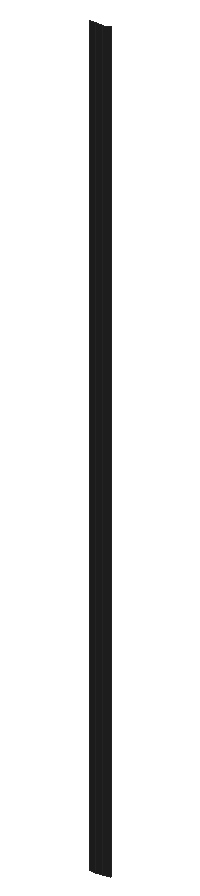
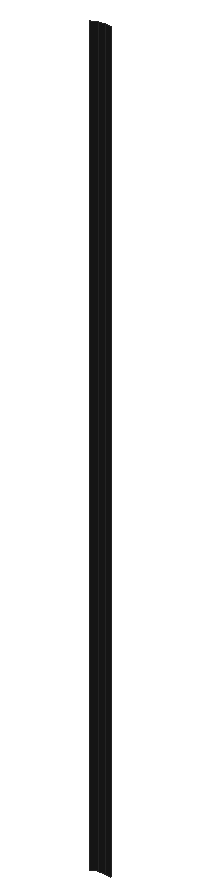
# SketchUp Ruby script. Lengths in inches.
U = 1.inch
M = Sketchup.active_model
def pt(a) = Geom::Point3d.new(a.map { |v| v * U })
def face(e, loops, mat)
  f = e.add_face(loops[0].map { |a| pt(a) })
  loops[1..].each { |l| e.add_face(l.map { |a| pt(a) }).erase! }
  f.material = f.back_material = mat if mat
  f
end
# faces: each face lists its corners as indices into pts; further lists are holes
def faces(e, pts, list, mat = nil) = list.each { |f| face(e, (f[0].is_a?(Array) ? f : [f]).map { |l| l.map { |i| pts[i] } }, mat) }
# xy, xz, yz: faces in a plane at the given z, y or x. An outline is a flat list of corners, or four numbers for a rectangle; further outlines are holes
def ring(l) = l.size == 4 ? [[l[0], l[1]], [l[2], l[1]], [l[2], l[3]], [l[0], l[3]]] : l.each_slice(2).to_a
def flat(e, list, mat, &to3) = list.each { |f| face(e, (f[0].is_a?(Array) ? f : [f]).map { |l| ring(l).map { |u, v| to3.(u, v) } }, mat) }
def xy(e, z, list, mat = nil) = flat(e, list, mat) { |x, y| [x, y, z] }
def xz(e, y, list, mat = nil) = flat(e, list, mat) { |x, z| [x, y, z] }
def yz(e, x, list, mat = nil) = flat(e, list, mat) { |y, z| [x, y, z] }
def lines(e, pts, list) = list.each { |a, b| e.add_line(pt(pts[a]), pt(pts[b])) }
# prism: a flat outline (further loops are holes) pulled along v
def prism(e, loops, v, mat = nil)
  f = face(e, loops, mat); d = Geom::Vector3d.new(v.map { |x| x * U })
  f.pushpull(f.normal.samedirection?(d) ? d.length : -d.length)
end
def box(e, o, s, mat = nil) = prism(e, [[o, [o[0] + s[0], o[1], o[2]], [o[0] + s[0], o[1] + s[1], o[2]], [o[0], o[1] + s[1], o[2]]]], [0, 0, s[2]], mat)
def at(x, y, z, deg = 0) = Geom::Transformation.translation(pt([x, y, z])) * Geom::Transformation.rotation(ORIGIN, Z_AXIS, deg.degrees)
def axes(o, x, y, z) = Geom::Transformation.new([*x, 0, *y, 0, *z, 0, *pt(o).to_a, 1])
def part(name) = M.definitions.add(name)
# library, detail: a bought-in or finely detailed component or shape, given as its bounding box
def library(name, o, s) = part(name).tap { |d| box(d.entities, o, s) }
def detail(e, o, s) = box(e.add_group.entities, o, s)
def put(e, d, t, mat = nil) = e.add_instance(d, t).tap { |i| i.material = mat if mat }
def group(e, t, mat = nil) = e.add_group.tap { |g| g.transformation = t; g.material = mat if mat }.entities
root = M.entities
M.materials.add("[0136_Charcoal]").color = [35, 35, 35]
p = [[263.28,227.52,142.6875],[263.52,227.49,142.6875],[263.52,227.49,171.3125],[263.28,227.52,171.3125],[263.76,227.52,142.6875],[263.76,227.52,171.3125],
  [263.99,227.61,142.6875],[263.99,227.61,171.3125]]
faces(root,p,[[0,1,2,3],[1,4,5,2],[4,6,7,5]],"[0136_Charcoal]")
